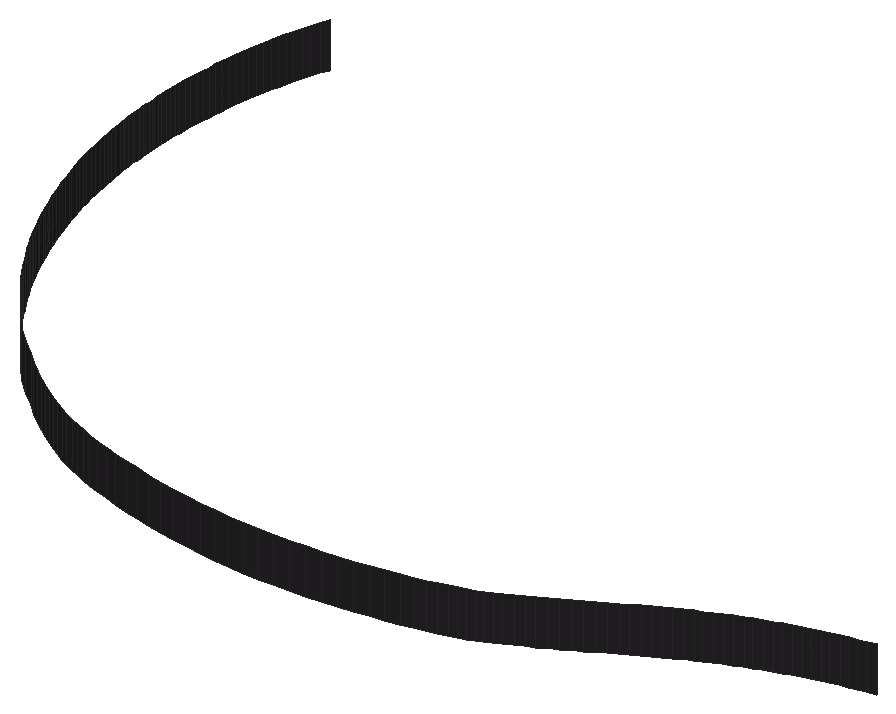
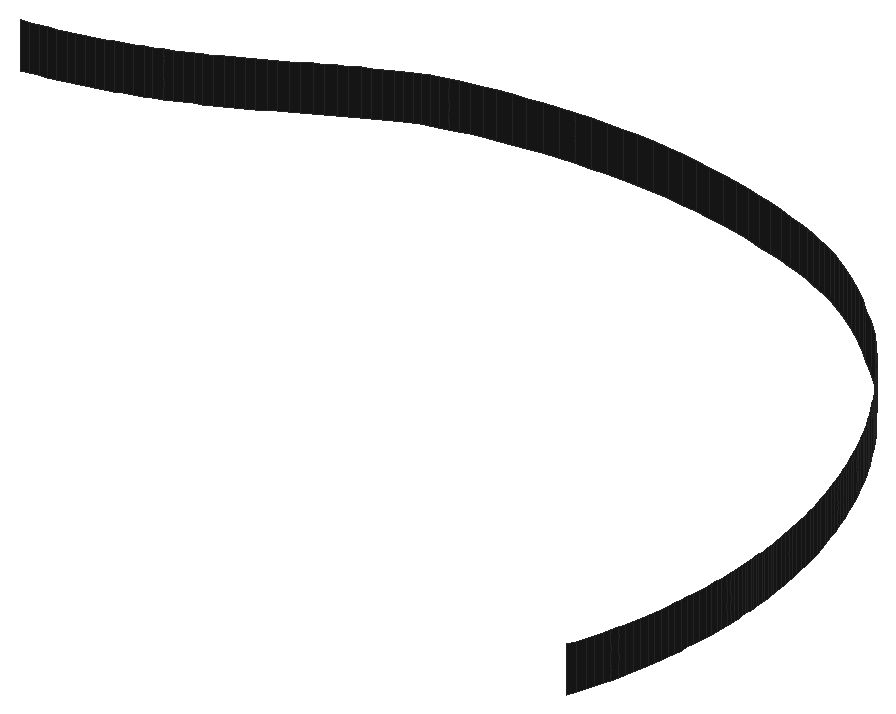
# SketchUp Ruby script. Lengths in inches.
U = 1.inch
M = Sketchup.active_model
def pt(a) = Geom::Point3d.new(a.map { |v| v * U })
def face(e, loops, mat)
  f = e.add_face(loops[0].map { |a| pt(a) })
  loops[1..].each { |l| e.add_face(l.map { |a| pt(a) }).erase! }
  f.material = f.back_material = mat if mat
  f
end
# faces: each face lists its corners as indices into pts; further lists are holes
def faces(e, pts, list, mat = nil) = list.each { |f| face(e, (f[0].is_a?(Array) ? f : [f]).map { |l| l.map { |i| pts[i] } }, mat) }
# xy, xz, yz: faces in a plane at the given z, y or x. An outline is a flat list of corners, or four numbers for a rectangle; further outlines are holes
def ring(l) = l.size == 4 ? [[l[0], l[1]], [l[2], l[1]], [l[2], l[3]], [l[0], l[3]]] : l.each_slice(2).to_a
def flat(e, list, mat, &to3) = list.each { |f| face(e, (f[0].is_a?(Array) ? f : [f]).map { |l| ring(l).map { |u, v| to3.(u, v) } }, mat) }
def xy(e, z, list, mat = nil) = flat(e, list, mat) { |x, y| [x, y, z] }
def xz(e, y, list, mat = nil) = flat(e, list, mat) { |x, z| [x, y, z] }
def yz(e, x, list, mat = nil) = flat(e, list, mat) { |y, z| [x, y, z] }
def lines(e, pts, list) = list.each { |a, b| e.add_line(pt(pts[a]), pt(pts[b])) }
# prism: a flat outline (further loops are holes) pulled along v
def prism(e, loops, v, mat = nil)
  f = face(e, loops, mat); d = Geom::Vector3d.new(v.map { |x| x * U })
  f.pushpull(f.normal.samedirection?(d) ? d.length : -d.length)
end
def box(e, o, s, mat = nil) = prism(e, [[o, [o[0] + s[0], o[1], o[2]], [o[0] + s[0], o[1] + s[1], o[2]], [o[0], o[1] + s[1], o[2]]]], [0, 0, s[2]], mat)
def at(x, y, z, deg = 0) = Geom::Transformation.translation(pt([x, y, z])) * Geom::Transformation.rotation(ORIGIN, Z_AXIS, deg.degrees)
def axes(o, x, y, z) = Geom::Transformation.new([*x, 0, *y, 0, *z, 0, *pt(o).to_a, 1])
def part(name) = M.definitions.add(name)
# library, detail: a bought-in or finely detailed component or shape, given as its bounding box
def library(name, o, s) = part(name).tap { |d| box(d.entities, o, s) }
def detail(e, o, s) = box(e.add_group.entities, o, s)
def put(e, d, t, mat = nil) = e.add_instance(d, t).tap { |i| i.material = mat if mat }
def group(e, t, mat = nil) = e.add_group.tap { |g| g.transformation = t; g.material = mat if mat }.entities
root = M.entities
M.materials.add("Marble_07_1K").color = [36, 34, 36]
xz(root,772.96,[[321.92,18,322.26,19],[322.26,18,322.59,19]],"Marble_07_1K")
yz(root,311.35,[[783.81,18,783.91,19],[783.91,18,784.02,19],[784.02,18,784.14,19],[784.14,18,784.27,19]],"Marble_07_1K")
yz(root,311.36,[[783.53,18,783.62,19],[783.62,18,783.71,19],[784.4,18,784.54,19]],"Marble_07_1K")
yz(root,311.37,[[783.36,18,783.45,19]],"Marble_07_1K")
yz(root,311.38,[[783.2,18,783.28,19]],"Marble_07_1K")
yz(root,311.39,[[783.03,18,783.12,19]],"Marble_07_1K")
p = [[320.58,773.08,18],[320.91,773.04,18],[320.91,773.04,19],[320.58,773.08,19],[321.25,773,18],[321.25,773,19],
  [321.58,772.98,18],[321.58,772.98,19],[321.92,772.96,18],[321.92,772.96,19],[322.59,772.96,18],[322.93,772.97,18],
  [322.93,772.97,19],[322.59,772.96,19],[323.27,772.99,18],[323.27,772.99,19],[323.6,773.02,18],[323.6,773.02,19],
  [323.93,773.05,18],[323.93,773.05,19],[319.91,773.1875,18],[320.24,773.13,18],[320.24,773.13,19],[319.91,773.1875,19],
  [324.26,773.09,18],[324.26,773.09,19],[324.57,773.14,18],[324.57,773.14,19],[324.87,773.1875,18],[324.87,773.1875,19],
  [319.59,773.25,18],[319.59,773.25,19],[325.15,773.24,18],[325.15,773.24,19],[325.42,773.29,18],[325.42,773.29,19],
  [318.97,773.4,18],[319.28,773.32,18],[319.28,773.32,19],[318.97,773.4,19],[325.65,773.35,18],[325.65,773.35,19],
  [325.87,773.4,18],[325.87,773.4,19],[318.68,773.47,18],[318.68,773.47,19],[326.05,773.45,18],[326.05,773.45,19],
  [326.23,773.5,18],[326.23,773.5,19],[318.41,773.55,18],[318.41,773.55,19],[326.39,773.55,18],[326.39,773.55,19],
  [317.92,773.71,18],[318.16,773.63,18],[318.16,773.63,19],[317.92,773.71,19],[326.54,773.61,18],[326.54,773.61,19],
  [326.68,773.67,18],[326.68,773.67,19],[317.71,773.79,18],[317.71,773.79,19],[326.83,773.74,18],[326.83,773.74,19],
  [326.99,773.8125,18],[326.99,773.8125,19],[317.51,773.87,18],[317.51,773.87,19],[327.15,773.9,18],[327.15,773.9,19],
  [317.32,773.96,18],[317.32,773.96,19],[327.32,773.99,18],[327.32,773.99,19],[316.96,774.14,18],[317.13,774.04,18],
  [317.13,774.04,19],[316.96,774.14,19],[327.5,774.08,18],[327.5,774.08,19],[316.78,774.24,18],[316.78,774.24,19],
  [327.68,774.18,18],[327.68,774.18,19],[316.61,774.34,18],[316.61,774.34,19],[327.87,774.28,18],[327.87,774.28,19],
  [316.43,774.46,18],[316.43,774.46,19],[328.05,774.39,18],[328.05,774.39,19],[328.24,774.49,18],[328.24,774.49,19],
  [316.24,774.59,18],[316.24,774.59,19],[328.42,774.6,18],[328.42,774.6,19],[316.03,774.74,18],[316.03,774.74,19],
  [328.6,774.7,18],[328.6,774.7,19],[315.81,774.9,18],[315.81,774.9,19],[328.77,774.8,18],[328.77,774.8,19],
  [328.9375,774.89,18],[328.9375,774.89,19],[315.57,775.1,18],[315.57,775.1,19],[329.1,774.99,18],[329.1,774.99,19],
  [329.27,775.08,18],[329.27,775.08,19],[315.3,775.33,18],[315.3,775.33,19],[329.43,775.17,18],[329.43,775.17,19],
  [329.59,775.25,18],[329.59,775.25,19],[314.99,775.59,18],[314.99,775.59,19],[329.75,775.34,18],[329.75,775.34,19],
  [329.92,775.42,18],[329.92,775.42,19],[330.08,775.49,18],[330.08,775.49,19],[330.24,775.57,18],[330.24,775.57,19],
  [314.66,775.89,18],[314.66,775.89,19],[330.4,775.64,18],[330.4,775.64,19],[330.57,775.71,18],[330.57,775.71,19],
  [330.74,775.78,18],[330.74,775.78,19],[330.9,775.84,18],[330.9,775.84,19],[331.07,775.91,18],[331.07,775.91,19],
  [314.36,776.24,18],[314.36,776.24,19],[331.24,775.97,18],[331.24,775.97,19],[331.41,776.02,18],[331.41,776.02,19],
  [331.58,776.08,18],[331.58,776.08,19],[331.75,776.13,18],[331.75,776.13,19],[331.92,776.18,18],[331.92,776.18,19],
  [314.11,776.54,18],[314.11,776.54,19],[332.09,776.23,18],[332.09,776.23,19],[332.26,776.27,18],[332.26,776.27,19],
  [332.4375,776.32,18],[332.4375,776.32,19],[332.61,776.36,18],[332.61,776.36,19],[332.79,776.39,18],[332.79,776.39,19],
  [332.96,776.43,18],[332.96,776.43,19],[333.14,776.46,18],[333.14,776.46,19],[313.89,776.82,18],[313.89,776.82,19],
  [313.7,777.0625,18],[313.7,777.0625,19],[313.54,777.28,18],[313.54,777.28,19],[313.4,777.48,18],[313.4,777.48,19],
  [313.27,777.67,18],[313.27,777.67,19],[313.16,777.84,18],[313.16,777.84,19],[313.06,778.01,18],[313.06,778.01,19],
  [312.96,778.17,18],[312.96,778.17,19],[312.87,778.32,18],[312.87,778.32,19],[312.78,778.47,18],[312.78,778.47,19],
  [312.7,778.62,18],[312.7,778.62,19],[312.63,778.77,18],[312.63,778.77,19],[312.56,778.91,18],[312.56,778.91,19],
  [312.49,779.05,18],[312.49,779.05,19],[312.42,779.2,18],[312.42,779.2,19],[312.35,779.35,18],[312.35,779.35,19],
  [312.29,779.49,18],[312.29,779.49,19],[312.23,779.64,18],[312.23,779.64,19],[312.17,779.79,18],[312.17,779.79,19],
  [312.11,779.94,18],[312.11,779.94,19],[312.05,780.09,18],[312.05,780.09,19],[312,780.24,18],[312,780.24,19],
  [311.95,780.39,18],[311.95,780.39,19],[311.9,780.55,18],[311.9,780.55,19],[311.85,780.7,18],[311.85,780.7,19],
  [311.81,780.85,18],[311.81,780.85,19],[311.76,781.01,18],[311.76,781.01,19],[311.72,781.16,18],[311.72,781.16,19],
  [311.68,781.32,18],[311.68,781.32,19],[311.65,781.47,18],[311.65,781.47,19],[311.61,781.63,18],[311.61,781.63,19],
  [311.58,781.79,18],[311.58,781.79,19],[311.55,781.9375,18],[311.55,781.9375,19],[311.52,782.09,18],[311.52,782.09,19],
  [311.5,782.23,18],[311.5,782.23,19],[311.48,782.37,18],[311.48,782.37,19],[311.46,782.5,18],[311.46,782.5,19],
  [311.4375,782.625,18],[311.4375,782.625,19],[311.42,782.74,18],[311.42,782.74,19],[311.41,782.84,18],[311.41,782.84,19],
  [311.4,782.9375,18],[311.4,782.9375,19],[311.39,783.03,18],[311.39,783.03,19],[311.38,783.2,18],[311.39,783.12,18],
  [311.39,783.12,19],[311.38,783.2,19],[311.37,783.36,18],[311.38,783.28,18],[311.38,783.28,19],[311.37,783.36,19],
  [311.36,783.53,18],[311.37,783.45,18],[311.37,783.45,19],[311.36,783.53,19],[311.35,783.81,18],[311.36,783.71,18],
  [311.36,783.71,19],[311.35,783.81,19],[311.36,784.4,18],[311.35,784.27,18],[311.35,784.27,19],[311.36,784.4,19],
  [311.37,784.6875,18],[311.36,784.54,18],[311.36,784.54,19],[311.37,784.6875,19],[311.38,784.84,18],[311.38,784.84,19],
  [311.39,784.99,18],[311.39,784.99,19],[311.41,785.15,18],[311.41,785.15,19],[311.42,785.3,18],[311.42,785.3,19],
  [311.44,785.46,18],[311.44,785.46,19],[311.46,785.62,18],[311.46,785.62,19],[311.48,785.78,18],[311.48,785.78,19],
  [311.51,785.9375,18],[311.51,785.9375,19],[311.54,786.09,18],[311.54,786.09,19],[311.56,786.25,18],[311.56,786.25,19],
  [311.6,786.41,18],[311.6,786.41,19],[311.63,786.57,18],[311.63,786.57,19],[311.67,786.73,18],[311.67,786.73,19],
  [311.71,786.89,18],[311.71,786.89,19],[311.75,787.05,18],[311.75,787.05,19],[311.8,787.22,18],[311.8,787.22,19],
  [311.86,787.39,18],[311.86,787.39,19],[311.92,787.57,18],[311.92,787.57,19],[311.99,787.75,18],[311.99,787.75,19]]
faces(root,p,[[0,1,2,3],[1,4,5,2],[4,6,7,5],[6,8,9,7],[10,11,12,13],[11,14,15,12],[14,16,17,15],[16,18,19,17],
  [20,21,22,23],[21,0,3,22],[18,24,25,19],[24,26,27,25],[26,28,29,27],[30,20,23,31],[28,32,33,29],[32,34,35,33],
  [36,37,38,39],[37,30,31,38],[34,40,41,35],[40,42,43,41],[44,36,39,45],[42,46,47,43],[46,48,49,47],[50,44,45,51],
  [48,52,53,49],[54,55,56,57],[55,50,51,56],[52,58,59,53],[58,60,61,59],[62,54,57,63],[60,64,65,61],[64,66,67,65],
  [68,62,63,69],[66,70,71,67],[72,68,69,73],[70,74,75,71],[76,77,78,79],[77,72,73,78],[74,80,81,75],[82,76,79,83],
  [80,84,85,81],[86,82,83,87],[84,88,89,85],[90,86,87,91],[88,92,93,89],[92,94,95,93],[96,90,91,97],[94,98,99,95],
  [100,96,97,101],[98,102,103,99],[104,100,101,105],[102,106,107,103],[106,108,109,107],[110,104,105,111],[108,112,113,109],[112,114,115,113],
  [116,110,111,117],[114,118,119,115],[118,120,121,119],[122,116,117,123],[120,124,125,121],[124,126,127,125],[126,128,129,127],[128,130,131,129],
  [132,122,123,133],[130,134,135,131],[134,136,137,135],[136,138,139,137],[138,140,141,139],[140,142,143,141],[144,132,133,145],[142,146,147,143],
  [146,148,149,147],[148,150,151,149],[150,152,153,151],[152,154,155,153],[156,144,145,157],[154,158,159,155],[158,160,161,159],[160,162,163,161],
  [162,164,165,163],[164,166,167,165],[166,168,169,167],[168,170,171,169],[172,156,157,173],[174,172,173,175],[176,174,175,177],[178,176,177,179],
  [180,178,179,181],[182,180,181,183],[184,182,183,185],[186,184,185,187],[188,186,187,189],[190,188,189,191],[192,190,191,193],[194,192,193,195],
  [196,194,195,197],[198,196,197,199],[200,198,199,201],[202,200,201,203],[204,202,203,205],[206,204,205,207],[208,206,207,209],[210,208,209,211],
  [212,210,211,213],[214,212,213,215],[216,214,215,217],[218,216,217,219],[220,218,219,221],[222,220,221,223],[224,222,223,225],[226,224,225,227],
  [228,226,227,229],[230,228,229,231],[232,230,231,233],[234,232,233,235],[236,234,235,237],[238,236,237,239],[240,238,239,241],[242,240,241,243],
  [244,242,243,245],[246,244,245,247],[248,246,247,249],[250,248,249,251],[252,250,251,253],[254,252,253,255],[256,257,258,259],[260,261,262,263],
  [264,265,266,267],[268,269,270,271],[272,273,274,275],[276,277,278,279],[280,276,279,281],[282,280,281,283],[284,282,283,285],[286,284,285,287],
  [288,286,287,289],[290,288,289,291],[292,290,291,293],[294,292,293,295],[296,294,295,297],[298,296,297,299],[300,298,299,301],[302,300,301,303],
  [304,302,303,305],[306,304,305,307],[308,306,307,309],[310,308,309,311],[312,310,311,313],[314,312,313,315],[316,314,315,317]],"Marble_07_1K")
